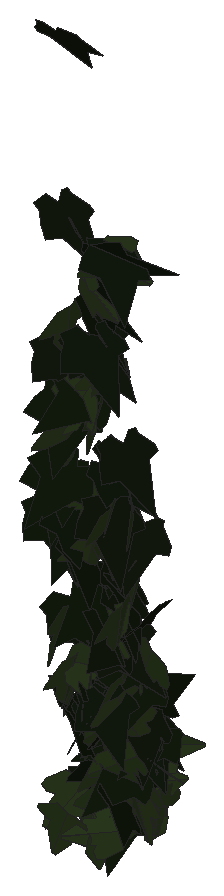
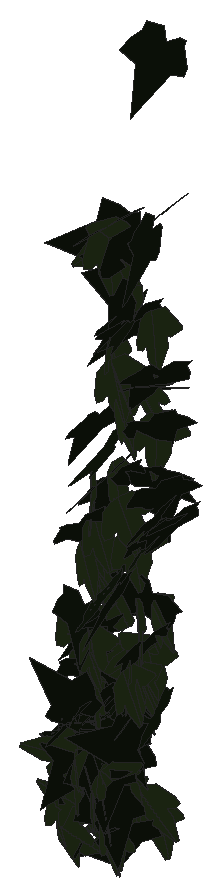
# SketchUp Ruby script. Lengths in inches.
U = 1.inch
M = Sketchup.active_model
def pt(a) = Geom::Point3d.new(a.map { |v| v * U })
def face(e, loops, mat)
  f = e.add_face(loops[0].map { |a| pt(a) })
  loops[1..].each { |l| e.add_face(l.map { |a| pt(a) }).erase! }
  f.material = f.back_material = mat if mat
  f
end
# faces: each face lists its corners as indices into pts; further lists are holes
def faces(e, pts, list, mat = nil) = list.each { |f| face(e, (f[0].is_a?(Array) ? f : [f]).map { |l| l.map { |i| pts[i] } }, mat) }
# xy, xz, yz: faces in a plane at the given z, y or x. An outline is a flat list of corners, or four numbers for a rectangle; further outlines are holes
def ring(l) = l.size == 4 ? [[l[0], l[1]], [l[2], l[1]], [l[2], l[3]], [l[0], l[3]]] : l.each_slice(2).to_a
def flat(e, list, mat, &to3) = list.each { |f| face(e, (f[0].is_a?(Array) ? f : [f]).map { |l| ring(l).map { |u, v| to3.(u, v) } }, mat) }
def xy(e, z, list, mat = nil) = flat(e, list, mat) { |x, y| [x, y, z] }
def xz(e, y, list, mat = nil) = flat(e, list, mat) { |x, z| [x, y, z] }
def yz(e, x, list, mat = nil) = flat(e, list, mat) { |y, z| [x, y, z] }
def lines(e, pts, list) = list.each { |a, b| e.add_line(pt(pts[a]), pt(pts[b])) }
# prism: a flat outline (further loops are holes) pulled along v
def prism(e, loops, v, mat = nil)
  f = face(e, loops, mat); d = Geom::Vector3d.new(v.map { |x| x * U })
  f.pushpull(f.normal.samedirection?(d) ? d.length : -d.length)
end
def box(e, o, s, mat = nil) = prism(e, [[o, [o[0] + s[0], o[1], o[2]], [o[0] + s[0], o[1] + s[1], o[2]], [o[0], o[1] + s[1], o[2]]]], [0, 0, s[2]], mat)
def at(x, y, z, deg = 0) = Geom::Transformation.translation(pt([x, y, z])) * Geom::Transformation.rotation(ORIGIN, Z_AXIS, deg.degrees)
def axes(o, x, y, z) = Geom::Transformation.new([*x, 0, *y, 0, *z, 0, *pt(o).to_a, 1])
def part(name) = M.definitions.add(name)
# library, detail: a bought-in or finely detailed component or shape, given as its bounding box
def library(name, o, s) = part(name).tap { |d| box(d.entities, o, s) }
def detail(e, o, s) = box(e.add_group.entities, o, s)
def put(e, d, t, mat = nil) = e.add_instance(d, t).tap { |i| i.material = mat if mat }
def group(e, t, mat = nil) = e.add_group.tap { |g| g.transformation = t; g.material = mat if mat }.entities
root = M.entities
M.materials.add("efeu1").color = [18, 25, 13]
M.materials.add("efeu2").color = [43, 57, 29]
c1 = part("ivyleaf_9")
p = [[1.54,2.16,1.25],[1.36,2.04,1.19],[-0.21,0.99,0.68],[-0.71,1.11,0.82],[-0.85,0.86,0.67],[-0.8,0.17,0.21],
  [-0.9,-0.01,0.1],[-0.67,-0.16,-0.02],[-0.08,-0.08,-0.05],[-0.03,-0.6,-0.4],[0.65,-0.88,-0.66],[0.83,-0.6,-0.49],
  [1.29,-0.42,-0.43],[1.8125,-0.07,-0.26],[1.21,0.44,0.15]]
faces(c1.entities,p,[[0,1,2,3,4,5,6,7,8,9,10,11,12,13,14]],"efeu1")
c2 = part("ivyleaf_10")
p = [[0,0.5,-0.03],[-0.0625,2.02,-0.43],[-0.19,2.01,-0.46],[-0.54,1.05,-0.29],[-0.52,0.625,-0.18],[-0.83,0.76,-0.28],
  [-1.16,0.64,-0.33],[-1.15,0.33,-0.24],[-0.77,-0.39,0.02],[-0.3,-0.51,0.16],[0.04,-0.48,0.23],[-0.02,2.01,-0.4375],
  [-0.06,2.01,-0.43],[0.04,-0.49,0.23],[0.67,-0.49,0.14],[1.38,0.36,-0.2],[1.375,0.51,-0.24],[0.81,0.65,-0.19],
  [0.62,0.59,-0.15],[0.6,1.09,-0.28],[0.5,1.23,-0.31]]
faces(c2.entities,p,[[0,1,2,3,4,5,6,7,8,9,10],[11,12,0,13,14,15,16,17,18,19,20]],"efeu2")
put(root,c1,axes([538.36,132.72,219.89],[-0.36832,-0.83408,-0.11414],[0.0331,0.11014,-0.91168],[0.8412,-0.36954,-0.0141]))
put(root,c1,axes([538.12,132.16,218.52],[0.1965,-0.84872,-0.33656],[0.01805,0.34781,-0.86655],[0.91284,0.17582,0.08959]))
put(root,c2,axes([538.9375,132.0625,206.47],[-0.77536,-0.11096,0.38201],[-0.37163,-0.09648,-0.78232],[0.14191,-0.85896,0.03852]))
put(root,c1,axes([538.35,134.48,206.86],[-0.19444,-0.76154,-0.32238],[0.09842,0.30751,-0.78577],[0.82109,-0.2172,0.01785]))
put(root,c2,axes([538.83,132.71,207.31],[0.81827,0.0334,-0.48662],[-0.48663,-0.00908,-0.8189],[-0.03335,0.95199,0.00927]))
put(root,c1,axes([538.53,132.07,237.52],[0.82774,0.39137,-0.32137],[-0.37146,0.05069,-0.89501],[-0.34419,0.88649,0.19306]))
put(root,c1,axes([538.11,132.94,210.97],[0.5793,-0.64432,0.10434],[0.0581,-0.08806,-0.86631],[0.65012,0.582,-0.01556]))
put(root,c1,axes([538.22,132.76,224.76],[0.03563,-0.79438,-0.5051],[0.16262,0.50305,-0.77969],[0.92721,-0.05771,0.15616]))
put(root,c2,axes([538.73,132.4,226.31],[-0.07606,-0.91791,-0.11043],[0.00995,0.10998,-0.92105],[0.92447,-0.07671,0.00082]))
put(root,c1,axes([538.57,132.83,222.57],[-0.48007,-0.79463,-0.12697],[0.07789,0.10127,-0.92828],[0.80093,-0.48614,0.01417]))
put(root,c2,axes([538.79,133.13,214.98],[0.51362,-0.58172,-0.4366],[-0.13836,0.44658,-0.75779],[0.71406,0.50497,0.16721]))
put(root,c2,axes([538.76,133.84,212.43],[-0.02012,-0.85394,0.19368],[0.01473,-0.19403,-0.85397],[0.87551,-0.01636,0.01882]))
put(root,c1,axes([538.92,132.49,220.21],[-0.80104,-0.44699,0.04924],[0.0024,-0.10484,-0.91263],[0.44969,-0.79567,0.09258]))
put(root,c1,axes([538.9,134.58,208.07],[0.39593,0.59622,-0.46108],[-0.2824,-0.36554,-0.71517],[-0.6988,0.48553,0.02777]))
put(root,c2,axes([538.95,134.61,208.82],[-0.39008,-0.47484,0.59059],[-0.11905,-0.6176,-0.57518],[0.7484,-0.34574,0.21633]))
put(root,c1,axes([538.39,133.35,214],[0.25094,-0.8063,-0.26613],[-0.01669,0.27278,-0.84216],[0.84892,0.24371,0.06212]))
put(root,c2,axes([538.74,132.96,212.08],[0.25287,-0.78851,0.29875],[0.11895,-0.27542,-0.82761],[0.83478,0.2781,0.02743]))
put(root,c2,axes([538.86,132.07,222.01],[-0.30458,-0.88809,-0.12991],[0.05164,0.11962,-0.93882],[0.89606,-0.30877,0.00995]))
put(root,c1,axes([538.65,132.91,217.95],[-0.24066,-0.8481,0.27912],[-0.01302,-0.28571,-0.87937],[0.89275,-0.23279,0.06242]))
put(root,c2,axes([538.76,132.11,214.46],[0.33125,-0.76683,0.30919],[0.11698,-0.28626,-0.8353],[0.8185,0.35125,-0.00575]))
put(root,c2,axes([538.88,134.71,206.91],[0.10256,-0.84329,-0.00153],[0.00221,0.00181,-0.8495],[0.84328,0.10256,0.00241]))
put(root,c1,axes([538.81,132.48,230],[0.72995,-0.05453,-0.60299],[-0.58438,0.18355,-0.72402],[0.15833,0.92883,0.10768]))
put(root,c2,axes([538.99,134.47,206.84],[0.02445,-0.84633,0.0904],[0.01218,-0.09008,-0.84663],[0.85106,0.0256,0.00952]))
put(root,c2,axes([539.07,132.125,212.64],[0.02711,-0.91946,-0.00946],[-0.00373,0.00935,-0.91986],[0.91951,0.02714,-0.00346]))
put(root,c2,axes([539.12,134.27,208.85],[-0.07755,-0.84578,0.03604],[-0.007,-0.03555,-0.84932],[0.84652,-0.07777,-0.00372]))
put(root,c1,axes([538.7,132.48,218.49],[0.14573,-0.88683,0.0445],[0.00368,-0.04449,-0.89871],[0.88793,0.14573,-0.00358]))
put(root,c2,axes([539.04,134.36,206.47],[0.57312,-0.60779,0.08293],[0.10096,-0.01848,-0.8332],[0.60505,0.5788,0.06047]))
put(root,c2,axes([539.1,134.52,207.47],[0.39988,-0.74958,0.06657],[0.07528,-0.03516,-0.84812],[0.74876,0.40386,0.04972]))
put(root,c1,axes([538.62,132.125,230.67],[0.46569,-0.80954,-0.25065],[0.08219,0.32779,-0.906],[0.84346,0.41502,0.22667]))
put(root,c2,axes([539.22,133.18,212.77],[0.43988,-0.64748,-0.40782],[-0.04518,0.4476,-0.75937],[0.76387,0.39933,0.18992]))
put(root,c1,axes([538.66,133.6,209.71],[0.42073,-0.02688,0.7568],[0.67268,0.41088,-0.35937],[-0.34779,0.76219,0.22043]))
put(root,c2,axes([539.09,134.46,206.58],[0.83898,-0.02794,0.02503],[0.02503,-0.00038,-0.83945],[0.02794,0.83935,0.00046]))
put(root,c1,axes([539.44,134.34,209.1875],[0.39264,0.67621,-0.34872],[-0.31772,-0.21084,-0.76657],[-0.69132,0.48095,0.15425]))
put(root,c1,axes([538.95,133.23,210.9375],[0.57653,-0.53226,-0.37239],[-0.1982,0.33003,-0.77856],[0.61862,0.60178,0.09761]))
put(root,c2,axes([539.625,134.7,207.64],[0.42467,-0.33661,0.74541],[-0.60238,0.4394,0.54161],[-0.55324,-0.73682,-0.01754]))
put(root,c2,axes([539.42,134.3,207.87],[0.34851,-0.73884,-0.28075],[-0.12221,0.25277,-0.81691],[0.78088,0.36931,-0.00255]))
put(root,c2,axes([539.38,134.53,208.02],[0.06521,-0.85643,-0.01203],[-0.00139,0.01196,-0.85891],[0.85652,0.06523,-0.00048]))
put(root,c2,axes([539.49,132.14,223.43],[0.86457,-0.23184,-0.3469],[-0.33755,0.0805,-0.89507],[0.24525,0.92809,-0.00902]))
put(root,c2,axes([539.45,133.29,218.94],[-0.35088,-0.78909,0.29764],[0.01011,-0.32629,-0.85311],[0.8433,-0.32441,0.13407]))
put(root,c1,axes([539.68,132.62,223.43],[-0.77108,-0.41641,0.31827],[-0.06849,-0.48124,-0.79559],[0.51962,-0.68136,0.36741]))
put(root,c2,axes([539.59,132.53,217.31],[-0.28224,-0.88714,0.06992],[-0.02141,-0.06656,-0.93095],[0.88963,-0.28305,-0.00023]))
put(root,c1,axes([539.1,133.1875,211.92],[0.52839,-0.68049,-0.18562],[-0.08594,0.16808,-0.86085],[0.70009,0.53423,0.03441]))
put(root,c1,axes([539.29,133.69,215.99],[0.50794,-0.53668,-0.55848],[-0.35203,0.43494,-0.73813],[0.68993,0.61704,0.03455]))
put(root,c1,axes([539.875,133.02,209.96],[-0.40785,0.68802,-0.30967],[0.12993,-0.28272,-0.79924],[-0.74323,-0.42697,0.03022]))
put(root,c2,axes([539.35,132.24,212.74],[0.10121,0.31723,0.83976],[0.18623,0.81928,-0.33193],[-0.87815,0.2103,0.02639]))
put(root,c2,axes([539.67,133.11,207.3],[-0.02391,-0.7945,0.37788],[0.05195,-0.37864,-0.7928],[0.87826,0.00076,0.05718]))
put(root,c1,axes([539.52,134.49,206.11],[-0.30807,-0.77862,-0.02139],[0.01369,0.01758,-0.83733],[0.7788,-0.30831,0.00626]))
put(root,c2,axes([539.68,133.01,222.71],[0.31684,-0.86275,0.11117],[0.02678,-0.10858,-0.91901],[0.86947,0.31773,-0.0122]))
put(root,c2,axes([539.8,133.48,207.76],[0.50058,-0.56773,-0.41231],[-0.16704,0.3955,-0.74738],[0.68148,0.51396,0.11967]))
put(root,c2,axes([539.65,132.48,210],[-0.03637,-0.1733,-0.89781],[0.17526,0.88054,-0.17706],[0.89743,-0.17898,-0.0018]))
put(root,c1,axes([539.16,132.46,210.04],[0.60282,-0.23133,-0.64445],[0.58365,-0.27534,0.64479],[-0.35802,-0.83838,-0.03394]))
put(root,c1,axes([539.08,132.19,215.22],[-0.02078,-0.44661,-0.91834],[0.72414,0.6412,-0.32821],[0.72002,-0.65776,0.30359]))
put(root,c2,axes([539.89,134.43,209.1875],[-0.33638,-0.78053,0.07618],[-0.01967,-0.07447,-0.84985],[0.78399,-0.33676,0.01137]))
put(root,c1,axes([539.3,132.44,216.93],[0.12599,-0.76384,0.51831],[0.25585,-0.47373,-0.76032],[0.88693,0.24516,0.1457]))
put(root,c1,axes([540.32,133.47,211.9],[-0.85606,0.07646,0.18632],[-0.18638,0.00756,-0.85943],[-0.07632,-0.87607,0.00884]))
put(root,c1,axes([539.35,132.9,226.53],[0.65216,-0.66483,-0.05791],[-0.02706,0.05456,-0.9311],[0.6668,0.65245,0.01886]))
put(root,c1,axes([540.09,132.54,211.63],[-0.58829,0.48867,-0.44066],[0.32337,-0.30009,-0.76449],[-0.57307,-0.67098,0.02098]))
put(root,c2,axes([540.35,132.8125,206.2],[-0.17489,0.14893,0.82216],[-0.51204,-0.68287,0.01478],[0.66026,-0.49013,0.22924]))
put(root,c2,axes([540.02,133.02,224.17],[-0.22053,-0.89404,0.11918],[-0.00054,-0.12256,-0.92039],[0.90195,-0.21867,0.02859]))
put(root,c1,axes([540.18,133.36,210.35],[0.08177,0.84621,0.05009],[-0.0851,0.05826,-0.84536],[-0.84341,0.07617,0.09015]))
put(root,c1,axes([540.15,132.51,208.95],[0.31966,0.86572,-0.27736],[-0.10387,-0.25729,-0.92282],[-0.90311,0.33602,0.00797]))
put(root,c2,axes([539.8,132.67,205.92],[0.07766,-0.28098,-0.83386],[0.36347,0.77259,-0.22648],[0.80135,-0.32319,0.18354]))
put(root,c2,axes([540.09,134.52,208.04],[0.0807,-0.85466,0.02079],[-0.00819,-0.02165,-0.8584],[0.85487,0.08047,-0.01019]))
put(root,c2,axes([540.05,132.82,208.76],[-0.29643,-0.76683,-0.36816],[0.10257,0.35481,-0.8216],[0.84442,-0.31229,-0.02945]))
put(root,c2,axes([540.7,134.79,206.28],[0.02234,-0.02076,-0.95461],[-0.83699,0.45911,-0.02957],[0.45952,0.83726,-0.00745]))
put(root,c1,axes([540.33,133.95,208.23],[0.24648,0.5613,-0.58767],[-0.24267,-0.53525,-0.61302],[-0.77558,0.34585,0.00504]))
put(root,c1,axes([540.6,133.96,209.5625],[-0.65599,-0.24274,0.48225],[-0.38211,-0.32739,-0.68456],[0.38142,-0.74546,0.14361]))
put(root,c2,axes([539.6,132.5625,227.7],[-0.33524,0.05692,-0.8855],[0.73885,-0.5063,-0.31226],[-0.49139,-0.8001,0.13461]))
put(root,c2,axes([540.1,132.71,223.99],[0.59458,-0.67331,0.27501],[0.1618,-0.22385,-0.89789],[0.70909,0.61566,-0.02571]))
put(root,c1,axes([539.73,134.11,215.53],[0.3446,-0.85266,0.25567],[0.12158,-0.2265,-0.91927],[0.88182,0.36444,0.02683]))
put(root,c2,axes([540.36,133.82,213.44],[0.0074,-0.89116,0.03833],[-0.00056,-0.03834,-0.89119],[0.89199,0.00736,-0.00088]))
put(root,c1,axes([539.81,132.21,225.87],[0.28193,-0.74172,-0.53908],[0.09419,0.58443,-0.75485],[0.91207,0.16891,0.24459]))
put(root,c2,axes([540.04,134.18,209.12],[0.74765,-0.37077,0.24795],[0.24931,-0.05394,-0.83239],[0.36986,0.78584,0.05985]))
put(root,c1,axes([540.0625,133.9,211.38],[-0.09763,-0.87575,0.11259],[-0.00618,-0.11259,-0.88115],[0.88294,-0.09762,0.00628]))
put(root,c1,axes([539.9,133.03,220.41],[0.58371,-0.50997,-0.4535],[-0.12283,0.5085,-0.72992],[0.6713,0.53647,0.26077]))
put(root,c2,axes([540.41,133.72,211.39],[0.62905,-0.54171,-0.29332],[-0.12847,0.29464,-0.81968],[0.60248,0.62843,0.13147]))
put(root,c2,axes([540.3,134.53,209.09],[0.24797,-0.79606,0.19306],[0.14209,-0.15685,-0.82926],[0.80671,0.27232,0.08673]))
put(root,c1,axes([540.04,133.03,211.47],[0.07103,-0.72276,-0.49697],[0.03588,0.50057,-0.72287],[0.87639,0.03808,0.06987]))
put(root,c2,axes([540.1875,134.6875,208.09],[0.84123,0.35034,0.16637],[0.1524,0.06679,-0.91126],[-0.35664,0.85492,0.00302]))
put(root,c2,axes([540.41,132.55,224.86],[0.22586,-0.89414,-0.1785],[0.13785,0.21527,-0.90389],[0.9013,0.19114,0.18298]))
put(root,c1,axes([540.12,131.92,226],[0.13098,-0.87528,-0.38354],[0.06799,0.39468,-0.87749],[0.95321,0.09212,0.1153]))
put(root,c2,axes([540.65,132.57,229.02],[-0.41699,-0.84809,0.02305],[0.00223,-0.02678,-0.94495],[0.8484,-0.41676,0.01382]))
put(root,c2,axes([540.62,133.23,217.86],[-0.08415,-0.88315,0.16431],[0.01284,-0.16619,-0.88671],[0.89821,-0.08036,0.02807]))
put(root,c2,axes([540.58,133.02,212.72],[-0.81365,-0.32982,-0.16392],[0.1562,0.05098,-0.87789],[0.33355,-0.82843,0.01124]))
put(root,c1,axes([539.84,132.52,227.4],[0.35083,0.07038,-0.88332],[0.87029,0.15141,0.35772],[0.16675,-0.9383,-0.00853]))
put(root,c2,axes([540.6875,132.93,212.22],[-0.04401,-0.80556,-0.36166],[0.02948,0.36057,-0.80672],[0.88253,-0.05222,0.00892]))
put(root,c1,axes([540.21,133.63,215.27],[0.26299,-0.84001,0.1609],[0.04084,-0.15581,-0.88019],[0.85431,0.26604,-0.00746]))
put(root,c1,axes([540.41,134.24,209.23],[0.69203,0.50832,0.0779],[0.07384,0.03102,-0.85846],[-0.50893,0.69571,-0.01864]))
put(root,c1,axes([540.18,132.94,221.13],[0.64151,-0.62842,-0.20152],[-0.05727,0.22697,-0.89009],[0.65745,0.63296,0.1191]))
put(root,c2,axes([540.14,132.53,214.1],[0.71634,-0.20374,-0.56691],[0.5395,-0.1749,0.74456],[-0.26801,-0.89662,-0.01642]))
put(root,c1,axes([540.97,133.77,209.76],[-0.79569,-0.29816,0.05171],[-0.04578,-0.02519,-0.84968],[0.29913,-0.79697,0.00751]))
put(root,c2,axes([540.69,132.73,208.23],[-0.35662,-0.73111,-0.3171],[0.13533,0.2868,-0.81344],[0.78534,-0.38142,-0.00382]))
put(root,c2,axes([540.86,131.83,219.23],[0.19991,-0.88318,-0.08378],[-0.00839,0.08399,-0.90547],[0.88711,0.19982,0.01031]))
put(root,c2,axes([541.42,132.35,209.66],[-0.44932,-0.21321,0.78121],[-0.71031,-0.32525,-0.4973],[0.38886,-0.84047,-0.00573]))
put(root,c2,axes([540.26,133.98,213.13],[0.4783,-0.25372,0.7536],[0.69752,-0.28837,-0.53979],[0.38178,0.84471,0.04208]))
put(root,c1,axes([540.68,132.64,214.125],[-0.26549,-0.5929,0.6501],[0.02199,-0.68331,-0.61421],[0.87959,-0.16187,0.21158]))
put(root,c1,axes([540.49,133.4,210.52],[0.26446,-0.84439,-0.0439],[-0.01605,0.04097,-0.88483],[0.84538,0.26493,-0.00307]))
put(root,c2,axes([540.43,132.22,229.21],[-0.41459,-0.40408,-0.76936],[0.69743,0.35383,-0.56166],[0.51844,-0.79912,0.14033]))
put(root,c1,axes([540.46,132.28,211.71],[-0.3228,-0.48529,-0.66571],[0.62509,0.32144,-0.53742],[0.5366,-0.66637,0.22558]))
put(root,c1,axes([541.17,133.3,214.43],[-0.02431,0.84008,0.20504],[-0.02078,0.20449,-0.84031],[-0.86449,-0.02854,0.01443]))
put(root,c2,axes([540.93,133.67,207.95],[-0.80584,0.31222,-0.04686],[0.04213,-0.02096,-0.8642],[-0.3129,-0.80693,0.00432]))
put(root,c1,axes([540.46,132.96,213.9375],[0.27637,-0.69901,-0.55122],[0.13349,0.60319,-0.69798],[0.88014,0.12801,0.27895]))
put(root,c2,axes([540.97,132.48,211.66],[-0.33769,-0.77554,-0.29308],[0.1166,0.26888,-0.84587],[0.82083,-0.35725,-0.00041]))
put(root,c2,axes([540.3,134.75,207.3],[0.27456,-0.04166,-0.80063],[0.79845,-0.0621,0.27705],[-0.07229,-0.84412,0.01913]))
put(root,c1,axes([540.21,132.26,229.02],[0.6841,-0.05676,0.67383],[0.67558,0.09884,-0.67756],[-0.02926,0.95513,0.11016]))
put(root,c2,axes([541.01,133.46,216.67],[0.2176,-0.87161,0.09066],[0.04609,-0.0819,-0.89803],[0.8751,0.22105,0.02475]))
put(root,c1,axes([540.72,132.24,219.27],[0.00301,-0.9132,-0.26924],[-0.0357,0.26895,-0.9126],[0.9514,0.01299,-0.0334]))
put(root,c2,axes([541.14,134.44,207.15],[-0.2208,-0.83333,-0.00911],[0.01288,0.00601,-0.86201],[0.83328,-0.2209,0.01091]))
put(root,c1,axes([540.94,133.75,218.1],[-0.30905,-0.83537,0.01129],[0.00013,-0.01208,-0.8907],[0.83545,-0.30902,0.00431]))
put(root,c1,axes([541.33,132.89,209.11],[-0.68744,-0.50128,0.24516],[-0.18565,-0.16139,-0.85055],[0.52623,-0.71178,0.0202]))
put(root,c2,axes([541.19,132.74,219.17],[0.4254,-0.58843,-0.54919],[-0.12238,0.56667,-0.70195],[0.79554,0.40182,0.18569]))
put(root,c1,axes([540.55,134.44,210.97],[-0.05545,-0.04098,0.85432],[0.77674,-0.36081,0.0331],[0.35806,0.77637,0.06048]))
put(root,c1,axes([541.13,133.47,212.39],[-0.47331,-0.7438,0.00341],[-0.00527,-0.00068,-0.88162],[0.74379,-0.47333,-0.00408]))
put(root,c2,axes([541.13,132.76,210.81],[-0.34852,-0.67984,-0.44514],[0.2075,0.39384,-0.76396],[0.78567,-0.40559,0.0043]))
put(root,c1,axes([540.46,133.65,209.15],[0.52066,-0.48003,0.49711],[0.52203,-0.13461,-0.67676],[0.4528,0.70717,0.20862]))
put(root,c2,axes([541.33,131.94,215.54],[0.08774,-0.89879,-0.16351],[-0.011,0.16321,-0.90305],[0.91347,0.0883,0.00483]))
put(root,c1,axes([541.32,134.35,209.91],[-0.59629,-0.57406,0.25472],[0.01488,-0.36406,-0.78564],[0.62786,-0.53657,0.26053]))
put(root,c1,axes([541.01,133.8,210.54],[-0.02703,-0.87017,0.04415],[0.01124,-0.04452,-0.8705],[0.87122,-0.02642,0.0126]))
put(root,c1,axes([540.93,134.13,210.25],[0.17576,-0.83791,-0.15723],[0.00111,0.16076,-0.85548],[0.85253,0.17254,0.03353]))
put(root,c1,axes([540.98,133.41,210.35],[0.18006,-0.78707,-0.35039],[0.02966,0.36341,-0.80108],[0.86103,0.15207,0.10087]))
put(root,c1,axes([540.92,132.27,229.44],[-0.0044,-0.94535,0.05301],[0.23693,-0.05243,-0.91523],[0.91672,0.00902,0.2368]))
put(root,c2,axes([541.3,133.0625,207.77],[-0.76299,0.31812,-0.17894],[0.13781,-0.13286,-0.82385],[-0.33798,-0.77235,0.06802]))
put(root,c1,axes([540.94,132.51,207.71],[0.09195,-0.65032,0.53623],[0.21136,-0.50439,-0.64795],[0.81596,0.20393,0.10741]))
put(root,c2,axes([541.81,133.15,213.4375],[-0.76541,0.19796,0.42981],[-0.44643,-0.03105,-0.78071],[-0.15691,-0.87728,0.12462]))
put(root,c2,axes([540.88,134.46,209.02],[-0.14791,-0.09482,0.84424],[0.64165,0.54917,0.17409],[-0.55679,0.65805,-0.02364]))
put(root,c1,axes([541.11,132.52,221.8125],[0.22509,-0.76528,-0.46033],[-0.07719,0.45628,-0.79629],[0.88972,0.23319,0.04737]))
